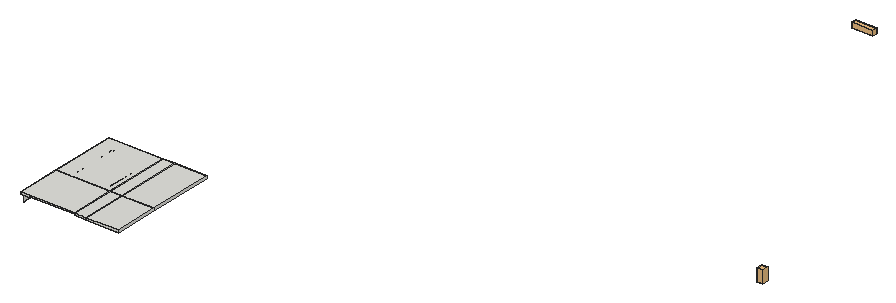
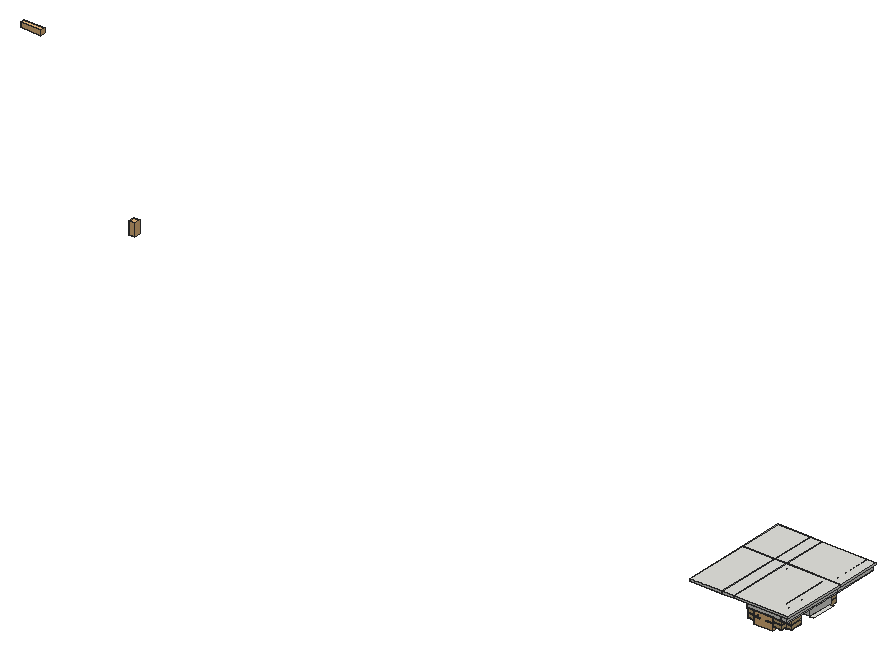
# SketchUp Ruby script. Lengths in inches.
U = 1.inch
M = Sketchup.active_model
def pt(a) = Geom::Point3d.new(a.map { |v| v * U })
def face(e, loops, mat)
  f = e.add_face(loops[0].map { |a| pt(a) })
  loops[1..].each { |l| e.add_face(l.map { |a| pt(a) }).erase! }
  f.material = f.back_material = mat if mat
  f
end
# faces: each face lists its corners as indices into pts; further lists are holes
def faces(e, pts, list, mat = nil) = list.each { |f| face(e, (f[0].is_a?(Array) ? f : [f]).map { |l| l.map { |i| pts[i] } }, mat) }
# xy, xz, yz: faces in a plane at the given z, y or x. An outline is a flat list of corners, or four numbers for a rectangle; further outlines are holes
def ring(l) = l.size == 4 ? [[l[0], l[1]], [l[2], l[1]], [l[2], l[3]], [l[0], l[3]]] : l.each_slice(2).to_a
def flat(e, list, mat, &to3) = list.each { |f| face(e, (f[0].is_a?(Array) ? f : [f]).map { |l| ring(l).map { |u, v| to3.(u, v) } }, mat) }
def xy(e, z, list, mat = nil) = flat(e, list, mat) { |x, y| [x, y, z] }
def xz(e, y, list, mat = nil) = flat(e, list, mat) { |x, z| [x, y, z] }
def yz(e, x, list, mat = nil) = flat(e, list, mat) { |y, z| [x, y, z] }
def lines(e, pts, list) = list.each { |a, b| e.add_line(pt(pts[a]), pt(pts[b])) }
# prism: a flat outline (further loops are holes) pulled along v
def prism(e, loops, v, mat = nil)
  f = face(e, loops, mat); d = Geom::Vector3d.new(v.map { |x| x * U })
  f.pushpull(f.normal.samedirection?(d) ? d.length : -d.length)
end
def box(e, o, s, mat = nil) = prism(e, [[o, [o[0] + s[0], o[1], o[2]], [o[0] + s[0], o[1] + s[1], o[2]], [o[0], o[1] + s[1], o[2]]]], [0, 0, s[2]], mat)
def at(x, y, z, deg = 0) = Geom::Transformation.translation(pt([x, y, z])) * Geom::Transformation.rotation(ORIGIN, Z_AXIS, deg.degrees)
def axes(o, x, y, z) = Geom::Transformation.new([*x, 0, *y, 0, *z, 0, *pt(o).to_a, 1])
def part(name) = M.definitions.add(name)
# library, detail: a bought-in or finely detailed component or shape, given as its bounding box
def library(name, o, s) = part(name).tap { |d| box(d.entities, o, s) }
def detail(e, o, s) = box(e.add_group.entities, o, s)
def put(e, d, t, mat = nil) = e.add_instance(d, t).tap { |i| i.material = mat if mat }
def group(e, t, mat = nil) = e.add_group.tap { |g| g.transformation = t; g.material = mat if mat }.entities
root = M.entities
M.materials.add("Emissive").color = [223, 214, 154]
M.materials.add("Generic").color = [208, 212, 208]
M.materials.add("Glass Safety 001").color = [0, 0, 0]
M.materials["Glass Safety 001"].alpha = 0.1
M.materials.add("Glass Tinted Gray").color = [0, 0, 0]
M.materials["Glass Tinted Gray"].alpha = 0.125
M.materials.add("[Color M08]").color = [30, 30, 30]
M.materials.add("[Wood Floor Light]").color = [204, 176, 127]
c1 = library("Chimney",[0,-14.34,0],[33.95,14.34,33.72])
c2 = library("Interior Props 221 031",[-3.74,-3.52,-0.04],[7.48,7.03,11.78])
c3 = library("Potted Plant 50-23",[-3.4,-3.5,0],[6.8,7,9.93])
c4 = part("Gruppo\#20")
prism(c4.entities,[[[0.51,10.14,0],[0.39,11.02,0],[0.07,11.02,0],[0.07,11.42,0],[0.79,11.42,0],[0.91,10.47,0],[1.01,9.52,0],[1.08,8.57,0],[1.14,7.62,0],[1.17,6.66,0],[1.18,5.71,0],[1.17,4.75,0],[1.14,3.8,0],[1.08,2.85,0],[1.01,1.9,0],[0.91,0.95,0],[0.79,0,0],[0,0,0],[0,0.39,0],[0.39,0.39,0],[0.51,1.27,0],[0.61,2.16,0],[0.6875,3.04,0],[0.74,3.93,0],[0.78,4.82,0],[0.79,5.71,0],[0.78,6.6,0],[0.74,7.49,0],[0.6875,8.375,0],[0.61,9.26,0]]],[0,0,0.39])
c5 = part("Tlon Cubo 860 Ceiling 152 005")
xy(c5.entities,-3.04,[[-16.54,-16.54,-16.54,16.54,16.54,-16.54],[16.54,-16.54,-16.54,16.54,16.54,16.54]])
xy(c5.entities,0,[[-16.93,-16.93,16.93,-16.93,-16.93,16.93],[16.93,-16.93,16.93,16.93,-16.93,16.93]])
xz(c5.entities,-16.93,[[-16.93,-3.79,16.93,-3.79,-16.93,0],[16.93,-3.79,16.93,0,-16.93,0]])
xz(c5.entities,-16.3,[[-16.3,-3.66,-16.3,-3.24,16.3,-3.24],[-16.3,-3.66,16.3,-3.24,16.3,-3.66]])
xz(c5.entities,16.3,[[-16.3,-3.66,16.3,-3.24,-16.3,-3.24],[-16.3,-3.66,16.3,-3.66,16.3,-3.24]])
xz(c5.entities,16.93,[[-16.93,-3.79,-16.93,0,16.93,0],[-16.93,-3.79,16.93,0,16.93,-3.79]])
yz(c5.entities,-16.93,[[-16.93,-3.79,-16.93,0,16.93,0],[-16.93,-3.79,16.93,0,16.93,-3.79]])
yz(c5.entities,-16.3,[[-16.3,-3.66,16.3,-3.66,-16.3,-3.24],[16.3,-3.66,16.3,-3.24,-16.3,-3.24]])
yz(c5.entities,16.3,[[-16.3,-3.66,-16.3,-3.24,16.3,-3.66],[16.3,-3.66,-16.3,-3.24,16.3,-3.24]])
yz(c5.entities,16.93,[[-16.93,-3.79,16.93,-3.79,-16.93,0],[16.93,-3.79,16.93,0,-16.93,0]])
p = [[-16.93,-16.93,-3.79],[-16.93,16.93,-3.79],[-16.3,16.3,-3.66],[-16.3,-16.3,-3.66],[16.93,-16.93,-3.79],[16.3,-16.3,-3.66],
  [16.93,16.93,-3.79],[16.3,16.3,-3.66]]
faces(c5.entities,p,[[0,1,2],[2,3,0],[4,0,3],[3,5,4],[6,4,5],[5,7,6],[2,1,6],[6,7,2]])
c6 = library("Kitchen utensil holder",[1778.15,4.69,382.13],[15.74,16.64,32.98])
c7 = library("Kitchen canister set",[1635.93,353.61,973.29],[56.89,12.6,12.71])
xy(root,77.12,[[102.36,276.64,119.26,289.64]],"Glass Tinted Gray")
xy(root,77.32,[[12.32,122.64,25.32,143.53]],"Glass Safety 001")
xy(root,77.5625,[[12.32,242.875,25.32,275.64]],"Glass Tinted Gray")
xy(root,77.87,[[102.36,289.64,119.26,290.64]],"Emissive")
xy(root,78.07,[[11.32,122.64,12.32,143.53]],"Emissive")
xy(root,78.3125,[[11.32,242.875,12.32,275.64]],"Emissive")
xy(root,78.39,[[102.36,276.64,119.26,290.64]],"Glass Tinted Gray")
xy(root,78.41,[[11.32,122.64,25.32,143.53]],"Glass Safety 001")
xy(root,78.43,[[11.32,242.875,25.32,275.64]],"Glass Safety 001")
xy(root,78.7,[[26.32,276.64,48.83,289.64]],"Glass Tinted Gray")
xy(root,79.45,[[26.32,289.64,48.83,290.64]],"Emissive")
xy(root,79.9,[[26.32,276.64,48.83,290.64]],"Glass Tinted Gray")
xy(root,84.97,[[0.32,145.89,9.32,214.64]])
xy(root,86.75,[[9.32,144.53,25.32,215.6]],"[Wood Floor Light]")
xy(root,87.75,[[11.32,162.66,25.32,163.8125],[11.32,181.72,25.32,182.875],[11.32,199.28,25.32,200.4375]])
xy(root,87.75,[[11.32,145.53,25.32,162.66],[11.32,163.8125,25.32,181.72],[11.32,182.875,25.32,199.28],[11.32,200.4375,25.32,214.6]],"[Wood Floor Light]")
xy(root,87.92,[[49.83,279.26,66.66,291.64]])
xy(root,88,[[85.24,279.26,101.36,291.64]],"Glass Tinted Gray")
xy(root,88.67,[[49.83,291.64,66.66,292.64]],"Emissive")
xy(root,88.75,[[85.24,291.64,101.36,292.64]],"Emissive")
xy(root,88.9375,[[85.24,279.26,101.36,292.64]],"Glass Tinted Gray")
xy(root,89.1,[[49.83,279.26,66.66,292.64]],"Glass Tinted Gray")
xy(root,89.5,[[12.32,242.875,25.32,275.64]],"Glass Tinted Gray")
xy(root,89.62,[[102.36,276.64,119.26,289.64]],"Glass Tinted Gray")
xy(root,89.69,[[12.32,122.64,25.32,143.53]],"Glass Safety 001")
xy(root,90.25,[[11.32,242.875,12.32,275.64]],"Emissive")
xy(root,90.37,[[102.36,289.64,119.26,290.64]],"Emissive")
xy(root,90.37,[[11.32,242.875,25.32,275.64]],"Glass Safety 001")
xy(root,90.44,[[11.32,122.64,12.32,143.53]],"Emissive")
xy(root,90.51,[[26.32,276.64,48.83,289.64]],"Glass Tinted Gray")
xy(root,90.78,[[11.32,122.64,25.32,143.53]],"Glass Safety 001")
xy(root,90.89,[[102.36,276.64,119.26,290.64]],"Glass Tinted Gray")
xy(root,91.26,[[26.32,289.64,48.83,290.64]],"Emissive")
xy(root,91.71,[[26.32,276.64,48.83,290.64]],"Glass Tinted Gray")
xy(root,102.04,[[11.32,162.66,25.32,163.8125],[11.32,181.72,25.32,182.875],[11.32,199.28,25.32,200.4375]])
xy(root,102.04,[[12.32,122.64,25.32,143.53],[12.32,145.53,25.32,162.66],[12.32,163.8125,25.32,181.72],[12.32,182.875,25.32,199.28],[12.32,200.4375,25.32,214.6],
  [12.32,242.875,25.32,275.64],[26.32,276.64,48.83,289.64],[102.36,276.64,119.26,289.64]],"[Wood Floor Light]")
xy(root,102.79,[[11.32,122.64,12.32,143.53],[11.32,145.53,12.32,162.66],[11.32,163.8125,12.32,181.72],[11.32,182.875,12.32,199.28],[11.32,200.4375,12.32,214.6],
  [11.32,242.875,12.32,275.64],[26.32,289.64,48.83,290.64],[102.36,289.64,119.26,290.64]],"Emissive")
xy(root,103.04,[[9.32,121.64,25.32,144.53],[9.32,144.53,25.32,215.6],[9.32,215.6,25.32,276.64],[9.32,276.64,25.32,292.64],[25.32,276.64,49.83,292.64],
  [101.36,276.64,120.26,292.64]])
xy(root,103.04,[[49.83,276.64,101.36,291.64]],"[Wood Floor Light]")
xy(root,103.79,[[49.83,291.64,101.36,292.64]],"Emissive")
xy(root,104.0625,[[9.32,121.64,25.32,292.64],[25.32,276.64,120.26,292.64]])
xy(root,118.5625,[[9.32,121.64,25.32,292.64],[25.32,276.64,120.26,292.64]])
xy(root,120,[[0.32,0,9.32,121.64],[9.32,0,25.32,121.64],[148.26,0,180.32,121.64],[180.32,0,268.26,121.64],[0.32,121.64,9.32,301.64],
  [9.32,121.64,25.32,292.64],[[25.32,121.64,25.32,276.64,120.26,276.64,120.26,292.64,148.26,292.64,148.26,121.64],[40.38,136.69,133.21,261.58]],[148.26,121.64,180.32,292.64],[180.32,121.64,268.26,292.64],[25.32,276.64,120.26,292.64],
  [9.32,292.64,148.26,301.64],[148.26,292.64,180.32,301.64],[180.32,292.64,268.26,301.64]])
xy(root,123,[[25.32,0,148.26,121.64],[[25.32,121.64,148.26,121.64,148.26,292.64,120.26,292.64,120.26,276.64,25.32,276.64],[39.44,135.75,134.14,262.52]]])
xy(root,123,[[39.44,135.75,40.38,262.52],[40.38,135.75,134.14,136.69],[133.21,136.69,134.14,261.58],[40.38,261.58,134.14,262.52]],"Emissive")
xy(root,124,[[39.44,135.75,134.14,262.52]])
xy(root,126,[[0.32,0,148.26,121.64],[148.26,0,180.32,121.64],[180.32,0,268.26,121.64],[0.32,121.64,148.26,301.64],[148.26,121.64,180.32,301.64],
  [180.32,121.64,268.26,301.64]])
xz(root,0,[[0.32,120,25.32,120,25.32,123,148.26,123,148.26,126,0.32,126],[148.26,120,180.32,126],[180.32,120,268.26,126]])
xz(root,121.64,[[0.32,120,0.32,126,148.26,126,148.26,123,25.32,123,25.32,120],[25.32,120,148.26,123],[148.26,120,180.32,126],[180.32,120,268.26,126]])
xz(root,121.64,[[9.32,103.04,25.32,104.0625],[9.32,104.0625,25.32,118.5625],[9.32,118.5625,25.32,120]],"[Color M08]")
xz(root,122.64,[[12.32,77.32,12.32,78.07,11.32,78.07,11.32,78.41,25.32,78.41,25.32,77.32],[12.32,89.69,12.32,90.44,11.32,90.44,11.32,90.78,25.32,90.78,25.32,89.69]])
xz(root,122.64,[[11.32,78.41,11.32,90.44,12.32,90.44,12.32,89.69,25.32,89.69,25.32,78.41],[11.32,90.78,11.32,102.79,12.32,102.79,12.32,102.04,25.32,102.04,25.32,90.78]],"[Wood Floor Light]")
xz(root,135.75,[[39.44,123,134.14,124]],"Emissive")
xz(root,136.69,[[40.38,120,133.21,123]])
xz(root,143.53,[[12.32,77.32,25.32,77.32,25.32,78.41,11.32,78.41,11.32,78.07,12.32,78.07],[12.32,89.69,25.32,89.69,25.32,90.78,11.32,90.78,11.32,90.44,12.32,90.44]])
xz(root,143.53,[[11.32,78.41,25.32,78.41,25.32,89.69,12.32,89.69,12.32,90.44,11.32,90.44],[11.32,90.78,25.32,90.78,25.32,102.04,12.32,102.04,12.32,102.79,11.32,102.79]],"[Wood Floor Light]")
xz(root,144.53,[[9.32,86.75,25.32,103.04]])
xz(root,145.53,[[11.32,87.75,11.32,102.79,12.32,102.79,12.32,102.04,25.32,102.04,25.32,87.75]],"[Wood Floor Light]")
xz(root,162.66,[[11.32,102.04,12.32,102.79]],"Emissive")
xz(root,162.66,[[11.32,87.75,25.32,102.04]],"Glass Safety 001")
xz(root,163.8125,[[11.32,102.04,12.32,102.79]],"Emissive")
xz(root,163.8125,[[11.32,87.75,25.32,102.04]],"Glass Safety 001")
xz(root,181.72,[[11.32,102.04,12.32,102.79]],"Emissive")
xz(root,181.72,[[11.32,87.75,25.32,102.04]],"Glass Safety 001")
xz(root,182.875,[[11.32,102.04,12.32,102.79]],"Emissive")
xz(root,182.875,[[11.32,87.75,25.32,102.04]],"Glass Safety 001")
xz(root,199.28,[[11.32,102.04,12.32,102.79]],"Emissive")
xz(root,199.28,[[11.32,87.75,25.32,102.04]],"Glass Safety 001")
xz(root,200.4375,[[11.32,102.04,12.32,102.79]],"Emissive")
xz(root,200.4375,[[11.32,87.75,25.32,102.04]],"Glass Safety 001")
xz(root,214.6,[[11.32,87.75,25.32,87.75,25.32,102.04,12.32,102.04,12.32,102.79,11.32,102.79]],"[Wood Floor Light]")
xz(root,215.6,[[9.32,86.75,25.32,103.04]])
xz(root,242.875,[[12.32,77.5625,12.32,78.3125,11.32,78.3125,11.32,78.43,25.32,78.43,25.32,77.5625],[12.32,89.5,12.32,90.25,11.32,90.25,11.32,90.37,25.32,90.37,25.32,89.5]])
xz(root,242.875,[[11.32,78.43,11.32,90.25,12.32,90.25,12.32,89.5,25.32,89.5,25.32,78.43],[11.32,90.37,11.32,102.79,12.32,102.79,12.32,102.04,25.32,102.04,25.32,90.37]],"[Wood Floor Light]")
xz(root,261.58,[[40.38,120,133.21,123]])
xz(root,262.52,[[39.44,123,134.14,124]],"Emissive")
xz(root,275.64,[[12.32,77.5625,25.32,77.5625,25.32,78.43,11.32,78.43,11.32,78.3125,12.32,78.3125],[12.32,89.5,25.32,89.5,25.32,90.37,11.32,90.37,11.32,90.25,12.32,90.25]])
xz(root,275.64,[[11.32,78.43,25.32,78.43,25.32,89.5,12.32,89.5,12.32,90.25,11.32,90.25],[11.32,90.37,25.32,90.37,25.32,102.04,12.32,102.04,12.32,102.79,11.32,102.79]],"[Wood Floor Light]")
xz(root,276.64,[[25.32,120,120.26,123]])
xz(root,276.64,[[25.72,104.0625,49.06,118.5625],[49.46,104.0625,72.79,118.5625],[73.19,104.0625,96.53,118.5625],[96.93,104.0625,120.26,118.5625]],"Generic")
xz(root,276.64,[[102.36,77.12,119.26,78.39],[26.32,78.7,48.83,79.9],[102.36,89.62,119.26,90.89],[26.32,90.51,48.83,91.71]],"Glass Tinted Gray")
xz(root,276.64,[[25.32,103.04,120.26,104.0625],[25.32,104.0625,25.72,118.5625],[49.06,104.0625,49.46,118.5625],[72.79,104.0625,73.19,118.5625],[96.53,104.0625,96.93,118.5625],
  [25.32,118.5625,120.26,120]],"[Color M08]")
xz(root,279.26,[[49.83,87.92,66.66,89.1],[85.24,88,101.36,88.9375]],"[Color M08]")
xz(root,289.64,[[102.36,77.12,119.26,77.87],[26.32,78.7,48.83,79.45],[102.36,89.62,119.26,90.37],[26.32,90.51,48.83,91.26],[26.32,102.04,48.83,102.79],
  [102.36,102.04,119.26,102.79]],"Emissive")
xz(root,290.64,[[102.36,77.87,119.26,78.39],[26.32,79.45,48.83,79.9],[102.36,90.37,119.26,90.89],[26.32,91.26,48.83,91.71]])
xz(root,290.64,[[102.36,78.39,119.26,90.37],[26.32,79.9,48.83,91.26],[102.36,90.89,119.26,102.79],[26.32,91.71,48.83,102.79]],"[Wood Floor Light]")
xz(root,291.64,[[49.83,87.92,66.66,88.67],[85.24,88,101.36,88.75],[49.83,103.04,101.36,103.79]],"Emissive")
xz(root,292.64,[[49.83,88.67,66.66,89.1],[85.24,88.75,101.36,88.9375],[9.32,103.04,25.32,104.0625],[25.32,103.04,25.32,104.0625,120.26,104.0625,120.26,103.04,101.36,103.04,101.36,103.79,49.83,103.79,49.83,103.04],[9.32,104.0625,25.32,118.5625],
  [25.32,104.0625,120.26,118.5625],[9.32,118.5625,25.32,120],[25.32,118.5625,120.26,120],[120.26,120,148.26,123]])
xz(root,301.64,[[0.32,120,148.26,126],[148.26,120,180.32,126],[180.32,120,268.26,126]])
yz(root,0.32,[[0,120,121.64,126],[121.64,120,301.64,126]])
yz(root,9.32,[[144.53,86.75,215.6,103.04],[0,103.04,121.64,104.0625],[121.64,103.04,292.64,104.0625],[0,104.0625,121.64,118.5625],[121.64,104.0625,292.64,118.5625],
  [0,118.5625,121.64,120],[121.64,118.5625,292.64,120]])
yz(root,11.32,[[122.64,78.07,143.53,78.41],[242.875,78.3125,275.64,78.43],[162.66,87.75,163.8125,102.04],[181.72,87.75,182.875,102.04],[199.28,87.75,200.4375,102.04],
  [242.875,90.25,275.64,90.37],[122.64,90.44,143.53,90.78]])
yz(root,11.32,[[122.64,78.41,143.53,90.44],[242.875,78.43,275.64,90.25],[145.53,87.75,162.66,102.79],[163.8125,87.75,181.72,102.79],[182.875,87.75,199.28,102.79],
  [200.4375,87.75,214.6,102.79],[242.875,90.37,275.64,102.79],[122.64,90.78,143.53,102.79]],"[Wood Floor Light]")
yz(root,12.32,[[122.64,77.32,143.53,78.07],[242.875,77.5625,275.64,78.3125],[242.875,89.5,275.64,90.25],[122.64,89.69,143.53,90.44],[122.64,102.04,143.53,102.79],
  [145.53,102.04,162.66,102.79],[163.8125,102.04,181.72,102.79],[182.875,102.04,199.28,102.79],[200.4375,102.04,214.6,102.79],[242.875,102.04,275.64,102.79]],"Emissive")
yz(root,25.32,[[276.64,103.04,292.64,104.0625],[276.64,104.0625,292.64,118.5625],[276.64,118.5625,292.64,120],[0,120,121.64,123],[121.64,120,276.64,123]])
yz(root,25.32,[[122.04,104.0625,147.47,118.5625],[147.87,104.0625,173.3,118.5625],[173.7,104.0625,199.14,118.5625],[199.54,104.0625,224.97,118.5625],[225.37,104.0625,250.8,118.5625],
  [251.2,104.0625,276.64,118.5625]],"Generic")
yz(root,25.32,[[122.64,77.32,143.53,78.41],[122.64,89.69,143.53,90.78]],"Glass Safety 001")
yz(root,25.32,[[242.875,77.5625,275.64,78.43],[242.875,89.5,275.64,90.37]],"Glass Tinted Gray")
yz(root,25.32,[[[144.53,86.75,215.6,103.04],[145.53,87.75,214.6,102.04]],[162.66,87.75,163.8125,102.04],[181.72,87.75,182.875,102.04],[199.28,87.75,200.4375,102.04],[121.64,103.04,276.64,104.0625],
  [121.64,104.0625,122.04,118.5625],[147.47,104.0625,147.87,118.5625],[173.3,104.0625,173.7,118.5625],[199.14,104.0625,199.54,118.5625],[224.97,104.0625,225.37,118.5625],
  [250.8,104.0625,251.2,118.5625],[121.64,118.5625,276.64,120]],"[Color M08]")
yz(root,26.32,[[276.64,78.7,289.64,78.7,289.64,79.45,290.64,79.45,290.64,79.9,276.64,79.9],[276.64,90.51,289.64,90.51,289.64,91.26,290.64,91.26,290.64,91.71,276.64,91.71]])
yz(root,26.32,[[276.64,79.9,290.64,79.9,290.64,91.26,289.64,91.26,289.64,90.51,276.64,90.51],[276.64,91.71,290.64,91.71,290.64,102.79,289.64,102.79,289.64,102.04,276.64,102.04]],"[Wood Floor Light]")
yz(root,39.44,[[135.75,123,262.52,124]],"Emissive")
yz(root,40.38,[[136.69,120,261.58,123]])
yz(root,48.83,[[276.64,78.7,276.64,79.9,290.64,79.9,290.64,79.45,289.64,79.45,289.64,78.7],[276.64,90.51,276.64,91.71,290.64,91.71,290.64,91.26,289.64,91.26,289.64,90.51]])
yz(root,48.83,[[276.64,79.9,276.64,90.51,289.64,90.51,289.64,91.26,290.64,91.26,290.64,79.9],[276.64,91.71,276.64,102.04,289.64,102.04,289.64,102.79,290.64,102.79,290.64,91.71]],"[Wood Floor Light]")
yz(root,49.83,[[279.26,87.92,291.64,87.92,291.64,88.67,292.64,88.67,292.64,89.1,279.26,89.1]])
yz(root,49.83,[[291.64,103.04,292.64,103.79]],"Emissive")
yz(root,49.83,[[276.64,87.92,279.26,89.1],[276.64,89.1,292.64,103.04]],"[Wood Floor Light]")
yz(root,66.66,[[279.26,87.92,291.64,87.92,291.64,88.67,292.64,88.67,292.64,89.1,279.26,89.1]],"[Color M08]")
yz(root,85.24,[[279.26,88,279.26,88.9375,292.64,88.9375,292.64,88.75,291.64,88.75,291.64,88]],"[Color M08]")
yz(root,101.36,[[276.64,88,279.26,88.9375],[279.26,88,279.26,88.9375,292.64,88.9375,292.64,88.75,291.64,88.75,291.64,88]])
yz(root,101.36,[[291.64,103.04,292.64,103.79]],"Emissive")
yz(root,101.36,[[276.64,88.9375,292.64,103.04]],"[Color M08]")
yz(root,102.36,[[276.64,77.12,289.64,77.12,289.64,77.87,290.64,77.87,290.64,78.39,276.64,78.39],[276.64,89.62,289.64,89.62,289.64,90.37,290.64,90.37,290.64,90.89,276.64,90.89]])
yz(root,102.36,[[276.64,78.39,290.64,78.39,290.64,90.37,289.64,90.37,289.64,89.62,276.64,89.62],[276.64,90.89,290.64,90.89,290.64,102.79,289.64,102.79,289.64,102.04,276.64,102.04]],"[Wood Floor Light]")
yz(root,119.26,[[276.64,77.12,276.64,78.39,290.64,78.39,290.64,77.87,289.64,77.87,289.64,77.12],[276.64,89.62,276.64,90.89,290.64,90.89,290.64,90.37,289.64,90.37,289.64,89.62]])
yz(root,119.26,[[276.64,78.39,276.64,89.62,289.64,89.62,289.64,90.37,290.64,90.37,290.64,78.39],[276.64,90.89,276.64,102.04,289.64,102.04,289.64,102.79,290.64,102.79,290.64,90.89]],"[Wood Floor Light]")
yz(root,120.26,[[276.64,120,292.64,123]])
yz(root,120.26,[[276.64,104.0625,292.64,118.5625],[276.64,118.5625,292.64,120]],"Generic")
yz(root,120.26,[[276.64,103.04,292.64,104.0625]],"[Color M08]")
yz(root,133.21,[[136.69,120,261.58,123]])
yz(root,134.14,[[135.75,123,262.52,124]],"Emissive")
yz(root,148.26,[[0,120,121.64,123],[121.64,120,292.64,123],[292.64,120,292.64,123,121.64,123,121.64,126,301.64,126,301.64,120],[0,123,121.64,126]])
yz(root,180.32,[[0,120,121.64,126],[121.64,120,301.64,126]])
yz(root,268.26,[[0,120,121.64,126],[121.64,120,301.64,126]])
p = [[66.66,290.9375,89.78],[66.66,290.9375,89.1],[66.66,290.9375,89.01]]
lines(root,p,[[0,1],[1,2]])
put(root,c1,axes([51.19,290.97,69.32],[1.4484,0,0],[0,1.33,0],[0,0,1]))
put(root,c2,at(21.78,130.94,78.41))
put(root,c3,at(95.22,284.77,88.9375))
put(root,c3,at(59.28,284.77,88.9375))
put(root,c3,at(17.73,131.93,90.78))
put(root,c4,axes([99.5,276.64,107.83],[0,-1,0],[0,0,0.6478],[-1,0,0]))
put(root,c4,axes([94.75,276.64,107.83],[0,-1,0],[0,0,0.6478],[-1,0,0]))
put(root,c4,axes([52.82,276.64,107.83],[0,-1,0],[0,0,0.6478],[-1,0,0]))
put(root,c4,axes([46.82,276.64,107.83],[0,-1,0],[0,0,0.6478],[-1,0,0]))
put(root,c4,axes([25.25,144.96,108.72],[1,0,0],[0,0,0.6478],[0,-1,0]))
put(root,c4,axes([25.25,149.64,108.72],[1,0,0],[0,0,0.6478],[0,-1,0]))
put(root,c4,axes([25.25,202.14,108.72],[1,0,0],[0,0,0.6478],[0,-1,0]))
put(root,c4,axes([25.25,197.46,108.72],[1,0,0],[0,0,0.6478],[0,-1,0]))
put(root,c4,axes([25.25,252.96,108.72],[1,0,0],[0,0,0.6478],[0,-1,0]))
put(root,c4,axes([25.25,248.27,108.72],[1,0,0],[0,0,0.6478],[0,-1,0]))
put(root,c5,axes([35.06,126.08,120.23],[0.11,0,0],[0,0.11,0],[0,0,0.11]))
put(root,c5,axes([35.06,154.14,120.23],[0.11,0,0],[0,0.11,0],[0,0,0.11]))
put(root,c5,axes([35.06,182.21,120.23],[0.11,0,0],[0,0.11,0],[0,0,0.11]))
put(root,c5,axes([35.06,210.27,120.23],[0.11,0,0],[0,0.11,0],[0,0,0.11]))
put(root,c5,axes([35.06,238.34,120.23],[0.11,0,0],[0,0.11,0],[0,0,0.11]))
put(root,c5,axes([35.06,266.4,120.23],[0.11,0,0],[0,0.11,0],[0,0,0.11]))
put(root,c5,axes([61.53,266.4,120.23],[0.11,0,0],[0,0.11,0],[0,0,0.11]))
put(root,c5,axes([88,266.4,120.23],[0.11,0,0],[0,0.11,0],[0,0,0.11]))
put(root,c5,axes([114.47,266.4,120.23],[0.11,0,0],[0,0.11,0],[0,0,0.11]))
put(root,c5,axes([140.93,266.4,120.23],[0.11,0,0],[0,0.11,0],[0,0,0.11]))
put(root,c5,axes([140.93,239.4375,120.23],[0.11,0,0],[0,0.11,0],[0,0,0.11]))
put(root,c5,axes([140.93,212.47,120.23],[0.11,0,0],[0,0.11,0],[0,0,0.11]))
put(root,c5,axes([140.93,185.51,120.23],[0.11,0,0],[0,0.11,0],[0,0,0.11]))
put(root,c5,axes([140.93,158.55,120.23],[0.11,0,0],[0,0.11,0],[0,0,0.11]))
put(root,c5,axes([140.93,131.59,120.23],[0.11,0,0],[0,0.11,0],[0,0,0.11]))
put(root,c5,axes([80.62,131.59,120.23],[0.11,0,0],[0,0.11,0],[0,0,0.11]))
put(root,c6,at(15.88,264.82,36))
put(root,c7,at(243.02,132.76,0))
